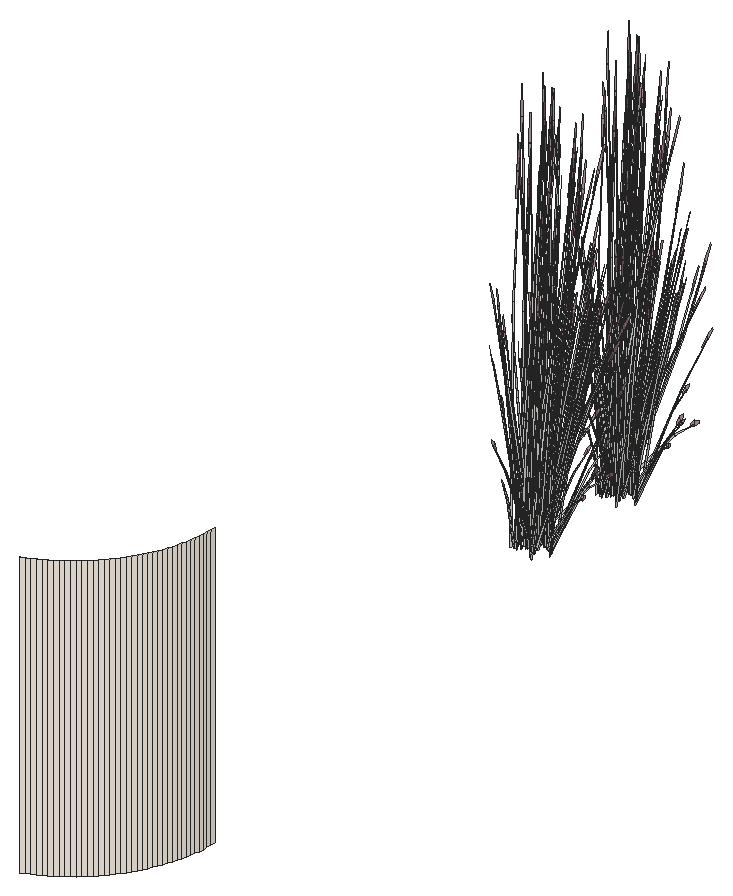
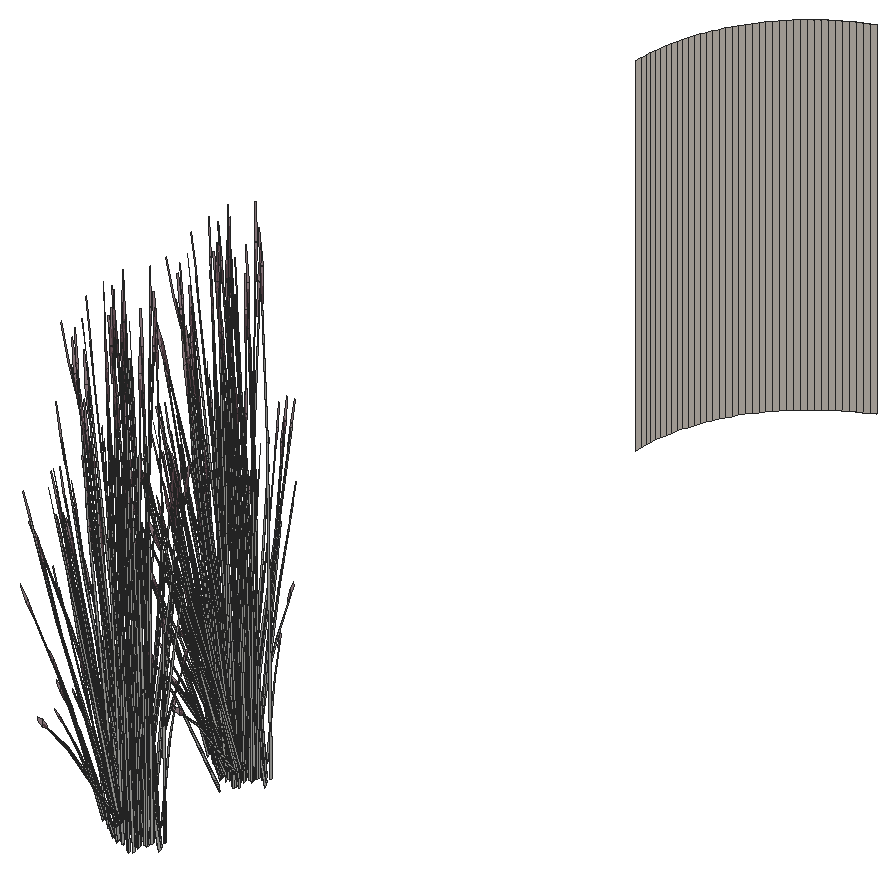
# SketchUp Ruby script. Lengths in inches.
U = 1.inch
M = Sketchup.active_model
def pt(a) = Geom::Point3d.new(a.map { |v| v * U })
def face(e, loops, mat)
  f = e.add_face(loops[0].map { |a| pt(a) })
  loops[1..].each { |l| e.add_face(l.map { |a| pt(a) }).erase! }
  f.material = f.back_material = mat if mat
  f
end
# faces: each face lists its corners as indices into pts; further lists are holes
def faces(e, pts, list, mat = nil) = list.each { |f| face(e, (f[0].is_a?(Array) ? f : [f]).map { |l| l.map { |i| pts[i] } }, mat) }
# xy, xz, yz: faces in a plane at the given z, y or x. An outline is a flat list of corners, or four numbers for a rectangle; further outlines are holes
def ring(l) = l.size == 4 ? [[l[0], l[1]], [l[2], l[1]], [l[2], l[3]], [l[0], l[3]]] : l.each_slice(2).to_a
def flat(e, list, mat, &to3) = list.each { |f| face(e, (f[0].is_a?(Array) ? f : [f]).map { |l| ring(l).map { |u, v| to3.(u, v) } }, mat) }
def xy(e, z, list, mat = nil) = flat(e, list, mat) { |x, y| [x, y, z] }
def xz(e, y, list, mat = nil) = flat(e, list, mat) { |x, z| [x, y, z] }
def yz(e, x, list, mat = nil) = flat(e, list, mat) { |y, z| [x, y, z] }
def lines(e, pts, list) = list.each { |a, b| e.add_line(pt(pts[a]), pt(pts[b])) }
# prism: a flat outline (further loops are holes) pulled along v
def prism(e, loops, v, mat = nil)
  f = face(e, loops, mat); d = Geom::Vector3d.new(v.map { |x| x * U })
  f.pushpull(f.normal.samedirection?(d) ? d.length : -d.length)
end
def box(e, o, s, mat = nil) = prism(e, [[o, [o[0] + s[0], o[1], o[2]], [o[0] + s[0], o[1] + s[1], o[2]], [o[0], o[1] + s[1], o[2]]]], [0, 0, s[2]], mat)
def at(x, y, z, deg = 0) = Geom::Transformation.translation(pt([x, y, z])) * Geom::Transformation.rotation(ORIGIN, Z_AXIS, deg.degrees)
def axes(o, x, y, z) = Geom::Transformation.new([*x, 0, *y, 0, *z, 0, *pt(o).to_a, 1])
def part(name) = M.definitions.add(name)
# library, detail: a bought-in or finely detailed component or shape, given as its bounding box
def library(name, o, s) = part(name).tap { |d| box(d.entities, o, s) }
def detail(e, o, s) = box(e.add_group.entities, o, s)
def put(e, d, t, mat = nil) = e.add_instance(d, t).tap { |i| i.material = mat if mat }
def group(e, t, mat = nil) = e.add_group.tap { |g| g.transformation = t; g.material = mat if mat }.entities
root = M.entities
M.materials.add("C01_Vanilla_Cream").color = [255, 246, 235]
M.materials.add("LightPink_Translucent").color = [144, 107, 117]
M.materials["LightPink_Translucent"].alpha = 0.75
c1 = part("blade")
p = [[2.15,0.21,22],[0,0.17,0],[0.09,0.45,0],[2.18,0.31,22],[2.29,0.31,22],[0.38,0.45,0],
  [2.48,0.24,33],[2.49,0.24,33],[2.48,0.22,33]]
faces(c1.entities,p,[[0,1,2,3],[4,5,2,3],[6,3,4,7],[8,0,3,6]])
c2 = part("seeds")
p = [[0.3,-0.1,1.38],[-0.01,-0.03,1.59],[-0.01,-0.03,0.03],[0.14,-0.07,-0.07],[0.29,-0.03,3],[0.15,0.01,3.11]]
faces(c2.entities,p,[[0,1,2,3],[1,0,4,5]],"LightPink_Translucent")
c3 = part("blade with seeds")
put(c3.entities,c1,at(0,0,0))
put(c3.entities,c2,axes([2.4,0.25,30.99],[1.5799,-0.05474,1.17369],[-0.12525,1.92788,0.29478],[-0.07173,-0.02425,1.56792]))
p = [[343.15,13.48,654],[342.625,13.26,654],[342.625,13.26,690],[343.15,13.48,690],[343.66,13.71,654],[343.66,13.71,690],
  [344.17,13.96,654],[344.17,13.96,690],[344.67,14.23,654],[344.67,14.23,690],[345.16,14.51,654],[345.16,14.51,690],
  [345.64,14.8,654],[345.64,14.8,690],[346.12,15.11,654],[346.12,15.11,690],[346.58,15.4375,654],[346.58,15.4375,690],
  [347.03,15.78,654],[347.03,15.78,690],[347.47,16.13,654],[347.47,16.13,690],[347.9,16.5,654],[347.9,16.5,690],
  [348.32,16.88,654],[348.32,16.88,690],[348.73,17.27,654],[348.73,17.27,690],[349.12,17.68,654],[349.12,17.68,690],
  [349.5,18.1,654],[349.5,18.1,690],[349.87,18.53,654],[349.87,18.53,690],[350.22,18.97,654],[350.22,18.97,690],
  [350.5625,19.42,654],[350.5625,19.42,690],[350.89,19.88,654],[350.89,19.88,690],[351.2,20.36,654],[351.2,20.36,690],
  [351.49,20.84,654],[351.49,20.84,690],[351.77,21.33,654],[351.77,21.33,690],[352.04,21.83,654],[352.04,21.83,690],
  [352.29,22.34,654],[352.29,22.34,690],[352.52,22.85,654],[352.52,22.85,690],[352.74,23.375,654],[352.74,23.375,690],
  [352.9375,23.9,654],[352.9375,23.9,690],[353.12,24.4375,654],[353.12,24.4375,690],[353.29,24.98,654],[353.29,24.98,690],
  [353.43,25.52,654],[353.43,25.52,690],[353.57,26.07,654],[353.57,26.07,690],[353.68,26.63,654],[353.68,26.63,690],
  [353.78,27.18,654],[353.78,27.18,690],[353.86,27.74,654],[353.86,27.74,690],[353.92,28.31,654],[353.92,28.31,690],
  [353.96,28.87,654],[353.96,28.87,690],[353.99,29.43,654],[353.99,29.43,690],[354,30,654],[354,30,690]]
faces(root,p,[[0,1,2,3],[4,0,3,5],[6,4,5,7],[8,6,7,9],[10,8,9,11],[12,10,11,13],[14,12,13,15],[16,14,15,17],
  [18,16,17,19],[20,18,19,21],[22,20,21,23],[24,22,23,25],[26,24,25,27],[28,26,27,29],[30,28,29,31],[32,30,31,33],
  [34,32,33,35],[36,34,35,37],[38,36,37,39],[40,38,39,41],[42,40,41,43],[44,42,43,45],[46,44,45,47],[48,46,47,49],
  [50,48,49,51],[52,50,51,53],[54,52,53,55],[56,54,55,57],[58,56,57,59],[60,58,59,61],[62,60,61,63],[64,62,63,65],
  [66,64,65,67],[68,66,67,69],[70,68,69,71],[72,70,71,73],[74,72,73,75],[76,74,75,77]],"C01_Vanilla_Cream")
put(root,c3,axes([343.01,92.84,656.125],[-0.14045,0.08385,1.17261],[-0.42064,-0.14676,-0.25218],[0.07797,-0.18252,0.50135]))
put(root,c3,axes([343.35,93.46,658.08],[0.01286,-0.38319,-0.58257],[0.54141,0.02574,0.0703],[0.05714,-0.16234,0.8241]))
put(root,c3,axes([344.11,92.86,657.87],[-0.00477,-0.08245,1.43454],[-0.40285,-0.23829,-0.22687],[0.06228,-0.14445,0.11505]))
put(root,c3,axes([342.74,93.27,657.18],[-0.092,0.14239,1.40529],[-0.38596,-0.29467,0.11363],[0.17411,-0.18366,0.60075]))
put(root,c3,axes([344,92.57,657.86],[-0.05018,0.03164,1.45454],[-0.49165,-0.10676,-0.13744],[-0.0178,-0.13809,0.2574]))
put(root,c3,axes([342.49,92.17,656.27],[0.06339,0.24157,0.94186],[-0.35163,-0.13379,0.69201],[0.03784,-0.12369,0.20745]))
put(root,c3,axes([343.24,93.33,657.84],[-0.35372,-0.27835,-0.41901],[0.37366,-0.24377,-0.32456],[0.05382,-0.14142,0.80174]))
put(root,c3,axes([342.47,92.92,657.88],[0.48688,0.1083,0.39362],[-0.16649,0.35605,0.32456],[-0.02926,-0.14002,0.8145]))
put(root,c3,axes([343.61,93.48,658.13],[-0.54305,-0.02053,-0.09971],[0.01484,-0.38862,-0.55346],[0.03772,-0.14967,0.84097]))
put(root,c3,axes([343.57,93.23,657.71],[0.33433,-0.21811,-0.29039],[0.31649,0.24905,0.3749],[0.04815,-0.12654,0.71734]))
put(root,c3,axes([342.6,92.89,657.88],[0.36409,-0.14079,0.05273],[0.17821,0.25674,0.41509],[-0.03516,-0.11317,0.63295]))
put(root,c3,axes([343.99,93.1,655.22],[-0.07396,-0.03263,1.44601],[-0.18997,-0.3646,-0.2209],[0.12815,-0.09894,0.2463]))
put(root,c3,axes([343.57,93.31,657.88],[0.35185,0.28265,0.39362],[-0.37366,0.24377,0.32456],[0.0649,-0.13261,0.8145]))
put(root,c3,axes([343.7,93.34,657.88],[0.40605,0.0193,0.05273],[-0.01113,0.29147,0.41509],[0.04249,-0.11165,0.63295]))
put(root,c3,axes([343.4,93.54,658.14],[-0.33433,0.21811,0.29039],[-0.31649,-0.24905,-0.3749],[0.04815,-0.12654,0.71734]))
put(root,c3,axes([343.99,94.125,658.08],[0.2581,-0.32687,-0.58257],[0.45228,0.2323,0.0703],[0.15411,-0.11843,0.8241]))
put(root,c3,axes([341.2,93.17,655.95],[-0.30893,-0.41511,0],[0.51685,-0.2315,-0.42318],[0.11772,-0.05273,1.34243]))
put(root,c3,axes([343.98,93.97,657.84],[-0.12693,-0.37826,-0.41901],[0.48071,-0.06617,-0.32456],[0.13776,-0.1016,0.80174]))
put(root,c3,axes([344.2,94.24,658.13],[-0.45707,-0.22842,-0.09971],[0.26332,-0.3308,-0.55346],[0.12913,-0.11499,0.84097]))
put(root,c3,axes([341.62,93.11,655.65],[0.46245,-0.20713,-0.40713],[0.27641,0.37142,0],[0.10533,-0.04718,1.29153]))
put(root,c3,axes([344.36,93.83,656.125],[-0.17652,-0.01227,1.17261],[-0.18084,-0.32916,-0.25218],[0.21685,-0.09312,0.50135]))
put(root,c3,axes([345.33,94.15,657.86],[-0.06454,-0.00315,1.45454],[-0.268,-0.33712,-0.13744],[0.10763,-0.11085,0.2574]))
put(root,c3,axes([342.17,93.96,655.6875],[0.33282,-0.31137,-0.51129],[0.41344,0.28235,-0.13419],[0.13336,-0.07767,1.12859]))
put(root,c3,axes([344.57,93.22,656.27],[-0.16458,0.21088,0.94186],[-0.14146,-0.28332,0.69201],[0.13593,-0.07099,0.20745]))
put(root,c3,axes([344.33,94.01,657.71],[0.43011,-0.0592,-0.29039],[0.11357,0.33844,0.3749],[0.12326,-0.0909,0.71734]))
put(root,c3,axes([341.81,94.32,656.1875],[-0.05758,-0.4727,-0.23858],[0.59969,-0.02858,-0.41002],[0.1056,-0.06296,1.3096]))
put(root,c3,axes([343.98,94.21,658.14],[-0.43011,0.0592,0.29039],[-0.11357,-0.33844,-0.3749],[0.12326,-0.0909,0.71734]))
put(root,c3,axes([341.73,93.27,655.66],[0.46099,0.1025,-0.25402],[-0.11607,0.36097,0.25402],[0.09293,-0.04163,1.13959]))
put(root,c3,axes([344.37,94.16,657.88],[0.33921,0.17422,0.05273],[-0.19749,0.2481,0.41509],[0.10876,-0.08021,0.63295]))
put(root,c3,axes([344.27,94.09,657.88],[0.12254,0.38127,0.39362],[-0.48071,0.06617,0.32456],[0.14168,-0.08967,0.8145]))
put(root,c3,axes([345.57,94.55,657.87],[0.06857,-0.0631,1.43454],[-0.08776,-0.38707,-0.22687],[0.17204,-0.07339,0.11505]))
put(root,c3,axes([341.88,94.69,656],[0.55674,0.20078,0.19733],[-0.26794,0.4172,0.41002],[0,-0.09617,1.31645]))
put(root,c3,axes([341.7,94.41,656.23],[-0.53657,0.02557,0.36686],[-0.04852,-0.4245,-0.17656],[0.09606,-0.04302,1.17788]))
put(root,c3,axes([344.22,95.14,658.13],[-0.24861,-0.37512,-0.09971],[0.44125,-0.18434,-0.55346],[0.18594,-0.04949,0.84097]))
put(root,c3,axes([344.2,94.8125,657.84],[0.13386,-0.37682,-0.41901],[0.45895,0.12916,-0.32456],[0.18478,-0.03455,0.80174]))
put(root,c3,axes([343.47,93.28,655.95],[0.30893,-0.41511,0],[0.51685,0.2315,-0.42318],[0.11772,0.05273,1.34243]))
put(root,c3,axes([344.6875,94.92,655.625],[-0.31825,0.04971,1.16098],[-0.05066,-0.39572,0.06645],[0.2229,-0.0599,0.66064]))
put(root,c3,axes([345.27,94.57,655.85],[-0.30634,-0.2649,-0.0532],[0.33551,-0.24272,-0.24121],[0.09507,-0.01709,0.7956]))
put(root,c3,axes([342.46,94.6,655.81],[0,-0.47933,0],[0.61786,0,0],[0,0,1.47154]))
put(root,c3,axes([343.21,93.5,656.03],[-0.46245,-0.20713,0.40713],[0.27641,-0.37142,0],[0.10533,0.04718,1.29153]))
put(root,c3,axes([344.11,94.95,658.08],[0.43419,-0.18296,-0.58257],[0.24197,0.37661,0.0703],[0.20979,-0.04278,0.8241]))
put(root,c3,axes([342.17,94.3,655.9375],[-0.40969,0.37595,0.37519],[-0.48673,-0.33186,0.14723],[0.09877,-0.03752,1.30262]))
put(root,c3,axes([341.45,93.68,656.03],[-0.14274,0.41171,0.14467],[-0.52234,-0.11651,0.28771],[0.09023,-0.00201,1.31534]))
put(root,c3,axes([344.05,95.02,658.14],[-0.41064,-0.11557,0.29039],[0.11977,-0.33716,-0.3749],[0.16533,-0.03092,0.71734]))
put(root,c3,axes([341.24,94.02,655.31],[-0.48636,0.16585,1.05721],[-0.1548,-0.47588,0.41079],[0.29865,0.00792,1.20246]))
put(root,c3,axes([342.54,94.14,656.15],[0.09532,-0.36971,0.11873],[0.46572,0.06418,-0.33905],[0.08476,0.03796,1.0393]))
put(root,c3,axes([345.04,94.66,655.22],[-0.02582,-0.06289,1.44601],[0.17911,-0.36789,-0.2209],[0.18067,-0.00529,0.2463]))
put(root,c3,axes([342.35,94.24,656.23],[-0.29683,-0.34771,0.36686],[0.44961,-0.24485,-0.17656],[0.09606,0.04302,1.17788]))
put(root,c3,axes([342.5,94.26,656.1875],[0.49889,-0.27503,-0.23858],[0.33175,0.38862,-0.41002],[0.12309,0.03947,1.3096]))
put(root,c3,axes([344.48,94.99,657.71],[0.41064,0.11557,-0.29039],[-0.11977,0.33716,0.3749],[0.16533,-0.03092,0.71734]))
put(root,c3,axes([343.75,93.53,655.65],[0.46245,0.20713,-0.40713],[-0.27641,0.37142,0],[0.10533,0.04718,1.29153]))
put(root,c3,axes([342.88,94.71,655.81],[0.55282,0,0],[0,0.42888,0],[0,0,1.46294]))
put(root,c3,axes([343.03,93.71,656.03],[-0.53096,0.10995,0.14467],[-0.13111,-0.40919,0.28771],[0.04735,0.05962,1.31534]))
put(root,c3,axes([343.36,94.57,657.18],[-0.20495,0.00938,1.40529],[0.13596,-0.40664,0.11363],[0.29207,0.02515,0.60075]))
put(root,c3,axes([343.625,93.68,655.66],[0.11607,0.36097,-0.25402],[-0.46099,0.1025,0.25402],[0.09293,0.04163,1.13959]))
put(root,c3,axes([344.42,95.13,657.88],[0.18148,0.28246,0.05273],[-0.33093,0.13825,0.41509],[0.14588,-0.02728,0.63295]))
put(root,c3,axes([342.7,94.49,655.95],[-0.62452,-0.08728,0.40343],[0.1271,-0.49295,0.15831],[0.09127,0.0476,1.40067]))
put(root,c3,axes([344.39,95.03,657.88],[-0.1396,0.37772,0.39362],[-0.45895,-0.12916,0.32456],[0.18049,-0.0227,0.8145]))
put(root,c3,axes([342.8,95.66,655.79],[0.51876,-0.14056,-0.15742],[0.18228,0.40489,0.00007],[0.05726,-0.01554,1.42596]))
put(root,c3,axes([342.87,94.89,655.82],[0.34492,0.26758,0],[-0.34492,0.26758,0],[0,0,1.38798]))
put(root,c3,axes([343.8,94.78,656.03],[-0.38822,-0.30175,0.14467],[0.39123,-0.29268,0.28771],[-0.04288,0.06162,1.31534]))
put(root,c3,axes([343.08,94.32,655.6875],[0.514,0.06792,-0.51129],[-0.10846,0.41895,-0.13419],[0.15339,0.05076,1.12859]))
put(root,c3,axes([345.35,95.05,656.27],[-0.30529,0.06839,0.94186],[0.1437,-0.28265,0.69201],[0.16196,0.01934,0.20745]))
put(root,c3,axes([342.86,94.58,656.23],[0.23974,-0.37328,0.36686],[0.49814,0.17965,-0.17656],[0,0.08605,1.17788]))
put(root,c3,axes([345.21,96.25,657.86],[-0.04468,-0.03627,1.45454],[0.09773,-0.38875,-0.13744],[0.17599,-0.02484,0.2574]))
put(root,c3,axes([342.77,94.8,655.88],[0,0.4791,-0.04622],[-0.61786,0,0],[0,0.01506,1.47081]))
put(root,c3,axes([342.8125,94.46,655.8125],[0.29683,0.34771,-0.36686],[-0.44961,0.24485,0.17656],[0.09606,0.04302,1.17788]))
put(root,c3,axes([344.82,95.93,657.22],[-0.09457,-0.34824,-0.02863],[0.44699,-0.08006,-0.12982],[0.09334,0.02208,0.42819]))
put(root,c3,axes([343.66,95.92,658.13],[0.02646,-0.4213,-0.09971],[0.50094,0.01152,-0.55346],[0.19293,0.02926,0.84097]))
put(root,c3,axes([344.12,94.79,656.03],[0,-0.41426,0.40713],[0.55282,0,0],[0,0.09435,1.29153]))
put(root,c3,axes([343.07,94.67,656.15],[0.46037,-0.12081,0.11873],[0.16122,0.34498,-0.33905],[0,0.07592,1.0393]))
put(root,c3,axes([343.59,95.75,658.14],[-0.28114,-0.25937,0.29039],[0.32102,-0.24553,-0.3749],[0.16311,0.03736,0.71734]))
put(root,c3,axes([344.78,95.51,656.125],[-0.119,-0.10189,1.17261],[0.15483,-0.33705,-0.25218],[0.24077,0.04566,0.50135]))
put(root,c3,axes([342.65,95.88,655.81],[0.49814,0.18599,0],[-0.23974,0.38645,0],[0,0,1.43462]))
put(root,c3,axes([344.1,95.66,657.87],[0.106,-0.00701,1.43454],[0.29074,-0.32184,-0.22687],[0.18854,0.04248,0.11505]))
put(root,c3,axes([343.6875,95.71,658.08],[0.49394,0.00997,-0.58257],[-0.03317,0.42002,0.0703],[0.20925,0.04433,0.8241]))
put(root,c3,axes([342.47,95.72,655.88],[0.21483,0.47591,-0.0493],[-0.61383,0.16676,0],[0.0075,0.01662,1.41182]))
put(root,c3,axes([344.49,94.86,655.95],[0.61786,0,0],[0,0.463,-0.42318],[0,0.10545,1.34243]))
put(root,c3,axes([344.25,95.1,655.8],[-0.61756,-0.00331,-0.04081],[0,-0.463,0.40953],[-0.01941,0.1054,1.29849]))
put(root,c3,axes([342.91,94.7,656.1875],[0.55647,0.19766,-0.23858],[-0.26794,0.4172,-0.41002],[0.01749,0.10243,1.3096]))
put(root,c3,axes([343.98,95.89,657.71],[0.28114,0.25937,-0.29039],[-0.32102,0.24553,0.3749],[0.16311,0.03736,0.71734]))
put(root,c3,axes([344.12,95.17,655.66],[-0.34492,0.25847,-0.25402],[-0.34492,-0.25847,0.25402],[0,0.08325,1.13959]))
put(root,c3,axes([343.84,95.99,657.88],[-0.02488,0.31501,0.05273],[-0.3757,-0.00864,0.41509],[0.14392,0.03296,0.63295]))
put(root,c3,axes([343.875,95.88,657.88],[-0.36434,0.27297,0.39362],[-0.31422,-0.28988,0.32456],[0.17094,0.05035,0.8145]))
put(root,c3,axes([342.72,96.2,658.14],[-0.07631,-0.33368,0.29039],[0.43626,-0.08811,-0.3749],[0.11718,0.09562,0.71734]))
put(root,c3,axes([344.36,95.17,655.65],[0,0.41426,-0.40713],[-0.55282,0,0],[0,0.09435,1.29153]))
put(root,c3,axes([342.97,95.22,657.18],[-0.18354,-0.07137,1.40529],[0.37983,-0.29943,0.11363],[0.23673,0.13508,0.60075]))
put(root,c3,axes([343.01,94.28,657.67],[-0.42697,-0.21524,1.13392],[0.45084,-0.33512,0.48925],[0.13776,0.20196,1.09604]))
put(root,c3,axes([343.65,96.03,656.27],[-0.27821,-0.11912,0.94186],[0.35924,-0.12103,0.69201],[0.09689,0.10252,0.20745]))
put(root,c3,axes([342.68,96.375,658.13],[0.29444,-0.35459,-0.09971],[0.4264,0.20428,-0.55346],[0.14822,0.10018,0.84097]))
put(root,c3,axes([342.29,96.67,657.86],[0.00146,-0.05015,1.45454],[0.42344,-0.22127,-0.13744],[0.14708,0.07898,0.2574]))
put(root,c3,axes([343.73,96.48,655.22],[0.036,-0.05981,1.44601],[0.45322,-0.17614,-0.2209],[0.1374,0.09116,0.2463]))
put(root,c3,axes([343.13,95.12,655.72],[0.18118,0.37929,-0.56754],[-0.52191,0.1366,-0.14895],[0.02003,0.12844,1.25274]))
put(root,c3,axes([343.03,96.2,657.84],[0.48758,-0.09847,-0.41901],[0.08529,0.37293,-0.32456],[0.13096,0.10687,0.80174]))
put(root,c3,axes([341.67,96.25,658.14],[0.14896,-0.31857,0.29039],[0.4346,0.09292,-0.3749],[0.03985,0.12826,0.71734]))
put(root,c3,axes([343.7,96.58,656.1875],[-0.31686,-0.01299,0.86149],[0.20925,-0.27594,0.47565],[0.12517,0.09804,0.67577]))
put(root,c3,axes([342.79,96.5,657.88],[-0.22457,0.26316,0.05273],[-0.3198,-0.15321,0.41509],[0.10339,0.08437,0.63295]))
put(root,c3,axes([342.26,97.39,658.63],[0.34145,-0.23766,-0.0532],[0.31287,0.26029,-0.24121],[0.02203,0.07375,0.7956]))
put(root,c3,axes([342.88,96.43,657.88],[-0.49145,0.09507,0.39362],[-0.08529,-0.37293,0.32456],[0.11558,0.10991,0.8145]))
put(root,c3,axes([342.66,95.91,656.125],[0.00872,-0.13732,1.17261],[0.41669,-0.15339,-0.25218],[0.12863,0.16436,0.50135]))
put(root,c3,axes([341.53,96.39,658.13],[0.48353,-0.19287,-0.09971],[0.23761,0.34232,-0.55346],[0.0638,0.14425,0.84097]))
put(root,c3,axes([341.94,96.37,657.84],[0.48573,0.10385,-0.41901],[-0.16649,0.35605,-0.32456],[0.04454,0.14335,0.80174]))
put(root,c3,axes([342.22,95.64,657.18],[-0.11295,-0.13301,1.40529],[0.52192,-0.11198,0.11363],[0.11796,0.20881,0.60075]))
put(root,c3,axes([341.77,96.3,658.08],[0.23583,0.33684,-0.58257],[-0.48546,0.18772,0.0703],[0.05515,0.16275,0.8241]))
put(root,c3,axes([341.41,97.15,657.87],[0.06263,0.06671,1.43454],[0.50546,0.02621,-0.22687],[0.05083,0.14712,0.11505]))
put(root,c3,axes([343.01,106.4375,656.125],[-0.14045,0.08385,1.17261],[-0.42064,-0.14676,-0.25218],[0.07797,-0.18252,0.50135]))
put(root,c3,axes([343.35,107.06,658.08],[0.01286,-0.38319,-0.58257],[0.54141,0.02574,0.0703],[0.05714,-0.16234,0.8241]))
put(root,c3,axes([344.11,106.46,657.87],[-0.00477,-0.08245,1.43454],[-0.40285,-0.23829,-0.22687],[0.06228,-0.14445,0.11505]))
put(root,c3,axes([342.74,106.86,657.18],[-0.092,0.14239,1.40529],[-0.38596,-0.29467,0.11363],[0.17411,-0.18366,0.60075]))
put(root,c3,axes([344,106.16,657.86],[-0.05018,0.03164,1.45454],[-0.49165,-0.10676,-0.13744],[-0.0178,-0.13809,0.2574]))
put(root,c3,axes([342.49,105.77,656.27],[0.06339,0.24157,0.94186],[-0.35163,-0.13379,0.69201],[0.03784,-0.12369,0.20745]))
put(root,c3,axes([343.24,106.93,657.84],[-0.35372,-0.27835,-0.41901],[0.37366,-0.24377,-0.32456],[0.05382,-0.14142,0.80174]))
put(root,c3,axes([342.47,106.52,657.88],[0.48688,0.1083,0.39362],[-0.16649,0.35605,0.32456],[-0.02926,-0.14002,0.8145]))
put(root,c3,axes([343.61,107.08,658.13],[-0.54305,-0.02053,-0.09971],[0.01484,-0.38862,-0.55346],[0.03772,-0.14967,0.84097]))
put(root,c3,axes([343.57,106.83,657.71],[0.33433,-0.21811,-0.29039],[0.31649,0.24905,0.3749],[0.04815,-0.12654,0.71734]))
put(root,c3,axes([342.6,106.49,657.88],[0.36409,-0.14079,0.05273],[0.17821,0.25674,0.41509],[-0.03516,-0.11317,0.63295]))
put(root,c3,axes([343.99,106.7,655.22],[-0.07396,-0.03263,1.44601],[-0.18997,-0.3646,-0.2209],[0.12815,-0.09894,0.2463]))
put(root,c3,axes([343.57,106.91,657.88],[0.35185,0.28265,0.39362],[-0.37366,0.24377,0.32456],[0.0649,-0.13261,0.8145]))
put(root,c3,axes([343.7,106.94,657.88],[0.40605,0.0193,0.05273],[-0.01113,0.29147,0.41509],[0.04249,-0.11165,0.63295]))
put(root,c3,axes([343.4,107.14,658.14],[-0.33433,0.21811,0.29039],[-0.31649,-0.24905,-0.3749],[0.04815,-0.12654,0.71734]))
put(root,c3,axes([343.99,107.72,658.08],[0.2581,-0.32687,-0.58257],[0.45228,0.2323,0.0703],[0.15411,-0.11843,0.8241]))
put(root,c3,axes([341.2,106.77,655.95],[-0.30893,-0.41511,0],[0.51685,-0.2315,-0.42318],[0.11772,-0.05273,1.34243]))
put(root,c3,axes([343.98,107.57,657.84],[-0.12693,-0.37826,-0.41901],[0.48071,-0.06617,-0.32456],[0.13776,-0.1016,0.80174]))
put(root,c3,axes([344.2,107.84,658.13],[-0.45707,-0.22842,-0.09971],[0.26332,-0.3308,-0.55346],[0.12913,-0.11499,0.84097]))
put(root,c3,axes([341.62,106.71,655.65],[0.46245,-0.20713,-0.40713],[0.27641,0.37142,0],[0.10533,-0.04718,1.29153]))
put(root,c3,axes([344.36,107.42,656.125],[-0.17652,-0.01227,1.17261],[-0.18084,-0.32916,-0.25218],[0.21685,-0.09312,0.50135]))
put(root,c3,axes([345.33,107.74,657.86],[-0.06454,-0.00315,1.45454],[-0.268,-0.33712,-0.13744],[0.10763,-0.11085,0.2574]))
put(root,c3,axes([342.17,107.56,655.6875],[0.33282,-0.31137,-0.51129],[0.41344,0.28235,-0.13419],[0.13336,-0.07767,1.12859]))
put(root,c3,axes([344.57,106.82,656.27],[-0.16458,0.21088,0.94186],[-0.14146,-0.28332,0.69201],[0.13593,-0.07099,0.20745]))
put(root,c3,axes([344.33,107.61,657.71],[0.43011,-0.0592,-0.29039],[0.11357,0.33844,0.3749],[0.12326,-0.0909,0.71734]))
put(root,c3,axes([341.81,107.92,656.1875],[-0.05758,-0.4727,-0.23858],[0.59969,-0.02858,-0.41002],[0.1056,-0.06296,1.3096]))
put(root,c3,axes([343.98,107.8125,658.14],[-0.43011,0.0592,0.29039],[-0.11357,-0.33844,-0.3749],[0.12326,-0.0909,0.71734]))
put(root,c3,axes([341.73,106.87,655.66],[0.46099,0.1025,-0.25402],[-0.11607,0.36097,0.25402],[0.09293,-0.04163,1.13959]))
put(root,c3,axes([344.37,107.76,657.88],[0.33921,0.17422,0.05273],[-0.19749,0.2481,0.41509],[0.10876,-0.08021,0.63295]))
put(root,c3,axes([344.27,107.68,657.88],[0.12254,0.38127,0.39362],[-0.48071,0.06617,0.32456],[0.14168,-0.08967,0.8145]))
put(root,c3,axes([345.57,108.15,657.87],[0.06857,-0.0631,1.43454],[-0.08776,-0.38707,-0.22687],[0.17204,-0.07339,0.11505]))
put(root,c3,axes([341.88,108.29,656],[0.55674,0.20078,0.19733],[-0.26794,0.4172,0.41002],[0,-0.09617,1.31645]))
put(root,c3,axes([341.7,108.01,656.23],[-0.53657,0.02557,0.36686],[-0.04852,-0.4245,-0.17656],[0.09606,-0.04302,1.17788]))
put(root,c3,axes([344.22,108.73,658.13],[-0.24861,-0.37512,-0.09971],[0.44125,-0.18434,-0.55346],[0.18594,-0.04949,0.84097]))
put(root,c3,axes([344.2,108.41,657.84],[0.13386,-0.37682,-0.41901],[0.45895,0.12916,-0.32456],[0.18478,-0.03455,0.80174]))
put(root,c3,axes([343.47,106.88,655.95],[0.30893,-0.41511,0],[0.51685,0.2315,-0.42318],[0.11772,0.05273,1.34243]))
put(root,c3,axes([344.6875,108.52,655.625],[-0.31825,0.04971,1.16098],[-0.05066,-0.39572,0.06645],[0.2229,-0.0599,0.66064]))
put(root,c3,axes([345.27,108.17,655.85],[-0.30634,-0.2649,-0.0532],[0.33551,-0.24272,-0.24121],[0.09507,-0.01709,0.7956]))
put(root,c3,axes([342.46,108.2,655.81],[0,-0.47933,0],[0.61786,0,0],[0,0,1.47154]))
put(root,c3,axes([343.21,107.09,656.03],[-0.46245,-0.20713,0.40713],[0.27641,-0.37142,0],[0.10533,0.04718,1.29153]))
put(root,c3,axes([344.11,108.55,658.08],[0.43419,-0.18296,-0.58257],[0.24197,0.37661,0.0703],[0.20979,-0.04278,0.8241]))
put(root,c3,axes([342.17,107.9,655.9375],[-0.40969,0.37595,0.37519],[-0.48673,-0.33186,0.14723],[0.09877,-0.03752,1.30262]))
put(root,c3,axes([341.45,107.28,656.03],[-0.14274,0.41171,0.14467],[-0.52234,-0.11651,0.28771],[0.09023,-0.00201,1.31534]))
put(root,c3,axes([344.05,108.62,658.14],[-0.41064,-0.11557,0.29039],[0.11977,-0.33716,-0.3749],[0.16533,-0.03092,0.71734]))
put(root,c3,axes([341.24,107.61,655.31],[-0.48636,0.16585,1.05721],[-0.1548,-0.47588,0.41079],[0.29865,0.00792,1.20246]))
put(root,c3,axes([342.54,107.74,656.15],[0.09532,-0.36971,0.11873],[0.46572,0.06418,-0.33905],[0.08476,0.03796,1.0393]))
put(root,c3,axes([345.04,108.26,655.22],[-0.02582,-0.06289,1.44601],[0.17911,-0.36789,-0.2209],[0.18067,-0.00529,0.2463]))
put(root,c3,axes([342.35,107.84,656.23],[-0.29683,-0.34771,0.36686],[0.44961,-0.24485,-0.17656],[0.09606,0.04302,1.17788]))
put(root,c3,axes([342.5,107.86,656.1875],[0.49889,-0.27503,-0.23858],[0.33175,0.38862,-0.41002],[0.12309,0.03947,1.3096]))
put(root,c3,axes([344.48,108.58,657.71],[0.41064,0.11557,-0.29039],[-0.11977,0.33716,0.3749],[0.16533,-0.03092,0.71734]))
put(root,c3,axes([343.75,107.13,655.65],[0.46245,0.20713,-0.40713],[-0.27641,0.37142,0],[0.10533,0.04718,1.29153]))
put(root,c3,axes([342.88,108.31,655.81],[0.55282,0,0],[0,0.42888,0],[0,0,1.46294]))
put(root,c3,axes([343.03,107.3,656.03],[-0.53096,0.10995,0.14467],[-0.13111,-0.40919,0.28771],[0.04735,0.05962,1.31534]))
put(root,c3,axes([343.36,108.17,657.18],[-0.20495,0.00938,1.40529],[0.13596,-0.40664,0.11363],[0.29207,0.02515,0.60075]))
put(root,c3,axes([343.625,107.28,655.66],[0.11607,0.36097,-0.25402],[-0.46099,0.1025,0.25402],[0.09293,0.04163,1.13959]))
put(root,c3,axes([344.42,108.73,657.88],[0.18148,0.28246,0.05273],[-0.33093,0.13825,0.41509],[0.14588,-0.02728,0.63295]))
put(root,c3,axes([342.7,108.09,655.95],[-0.62452,-0.08728,0.40343],[0.1271,-0.49295,0.15831],[0.09127,0.0476,1.40067]))
put(root,c3,axes([344.39,108.625,657.88],[-0.1396,0.37772,0.39362],[-0.45895,-0.12916,0.32456],[0.18049,-0.0227,0.8145]))
put(root,c3,axes([342.8,109.26,655.79],[0.51876,-0.14056,-0.15742],[0.18228,0.40489,0.00007],[0.05726,-0.01554,1.42596]))
put(root,c3,axes([342.87,108.49,655.82],[0.34492,0.26758,0],[-0.34492,0.26758,0],[0,0,1.38798]))
put(root,c3,axes([343.8,108.375,656.03],[-0.38822,-0.30175,0.14467],[0.39123,-0.29268,0.28771],[-0.04288,0.06162,1.31534]))
put(root,c3,axes([343.08,107.92,655.6875],[0.514,0.06792,-0.51129],[-0.10846,0.41895,-0.13419],[0.15339,0.05076,1.12859]))
put(root,c3,axes([345.35,108.65,656.27],[-0.30529,0.06839,0.94186],[0.1437,-0.28265,0.69201],[0.16196,0.01934,0.20745]))
put(root,c3,axes([342.86,108.18,656.23],[0.23974,-0.37328,0.36686],[0.49814,0.17965,-0.17656],[0,0.08605,1.17788]))
put(root,c3,axes([345.21,109.85,657.86],[-0.04468,-0.03627,1.45454],[0.09773,-0.38875,-0.13744],[0.17599,-0.02484,0.2574]))
put(root,c3,axes([342.77,108.39,655.88],[0,0.4791,-0.04622],[-0.61786,0,0],[0,0.01506,1.47081]))
put(root,c3,axes([342.8125,108.05,655.8125],[0.29683,0.34771,-0.36686],[-0.44961,0.24485,0.17656],[0.09606,0.04302,1.17788]))
put(root,c3,axes([344.82,109.52,657.22],[-0.09457,-0.34824,-0.02863],[0.44699,-0.08006,-0.12982],[0.09334,0.02208,0.42819]))
put(root,c3,axes([343.66,109.51,658.13],[0.02646,-0.4213,-0.09971],[0.50094,0.01152,-0.55346],[0.19293,0.02926,0.84097]))
put(root,c3,axes([344.12,108.39,656.03],[0,-0.41426,0.40713],[0.55282,0,0],[0,0.09435,1.29153]))
put(root,c3,axes([343.07,108.27,656.15],[0.46037,-0.12081,0.11873],[0.16122,0.34498,-0.33905],[0,0.07592,1.0393]))
put(root,c3,axes([343.59,109.35,658.14],[-0.28114,-0.25937,0.29039],[0.32102,-0.24553,-0.3749],[0.16311,0.03736,0.71734]))
put(root,c3,axes([344.78,109.11,656.125],[-0.119,-0.10189,1.17261],[0.15483,-0.33705,-0.25218],[0.24077,0.04566,0.50135]))
put(root,c3,axes([342.65,109.48,655.81],[0.49814,0.18599,0],[-0.23974,0.38645,0],[0,0,1.43462]))
put(root,c3,axes([344.1,109.26,657.87],[0.106,-0.00701,1.43454],[0.29074,-0.32184,-0.22687],[0.18854,0.04248,0.11505]))
put(root,c3,axes([343.6875,109.3125,658.08],[0.49394,0.00997,-0.58257],[-0.03317,0.42002,0.0703],[0.20925,0.04433,0.8241]))
put(root,c3,axes([342.47,109.32,655.88],[0.21483,0.47591,-0.0493],[-0.61383,0.16676,0],[0.0075,0.01662,1.41182]))
put(root,c3,axes([344.49,108.46,655.95],[0.61786,0,0],[0,0.463,-0.42318],[0,0.10545,1.34243]))
put(root,c3,axes([344.25,108.7,655.8],[-0.61756,-0.00331,-0.04081],[0,-0.463,0.40953],[-0.01941,0.1054,1.29849]))
put(root,c3,axes([342.91,108.29,656.1875],[0.55647,0.19766,-0.23858],[-0.26794,0.4172,-0.41002],[0.01749,0.10243,1.3096]))
put(root,c3,axes([343.98,109.48,657.71],[0.28114,0.25937,-0.29039],[-0.32102,0.24553,0.3749],[0.16311,0.03736,0.71734]))
put(root,c3,axes([344.12,108.76,655.66],[-0.34492,0.25847,-0.25402],[-0.34492,-0.25847,0.25402],[0,0.08325,1.13959]))
put(root,c3,axes([343.84,109.58,657.88],[-0.02488,0.31501,0.05273],[-0.3757,-0.00864,0.41509],[0.14392,0.03296,0.63295]))
put(root,c3,axes([342.85,108.6,655.8125],[-0.23974,0.37328,-0.36686],[-0.49814,-0.17965,0.17656],[0,0.08605,1.17788]))
put(root,c3,axes([343.875,109.48,657.88],[-0.36434,0.27297,0.39362],[-0.31422,-0.28988,0.32456],[0.17094,0.05035,0.8145]))
